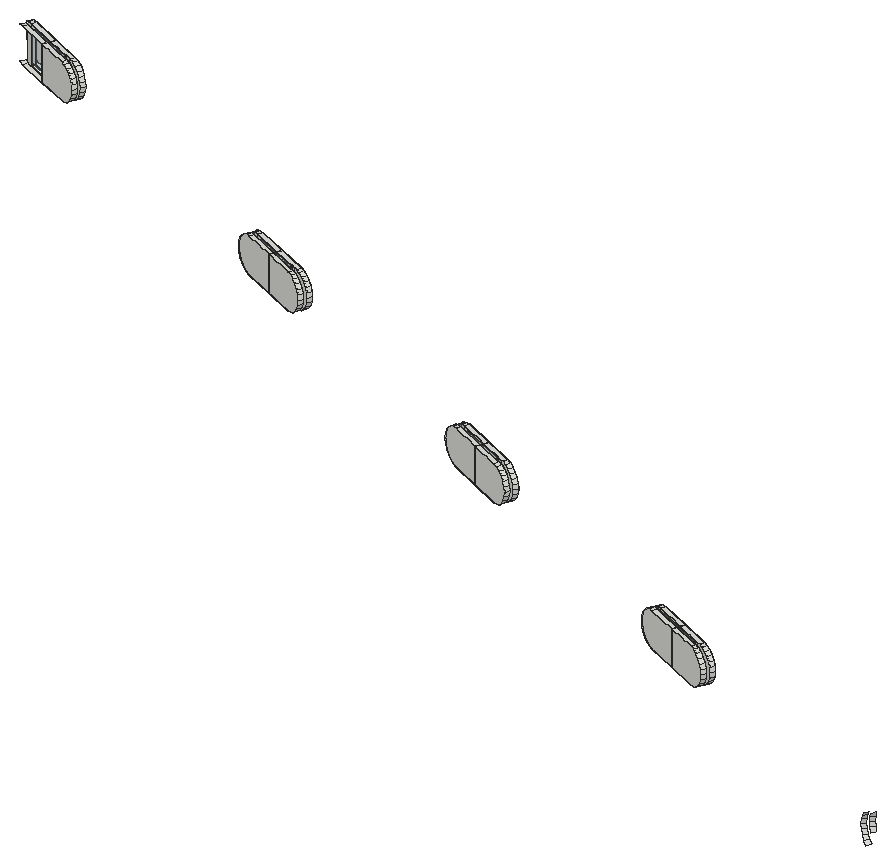
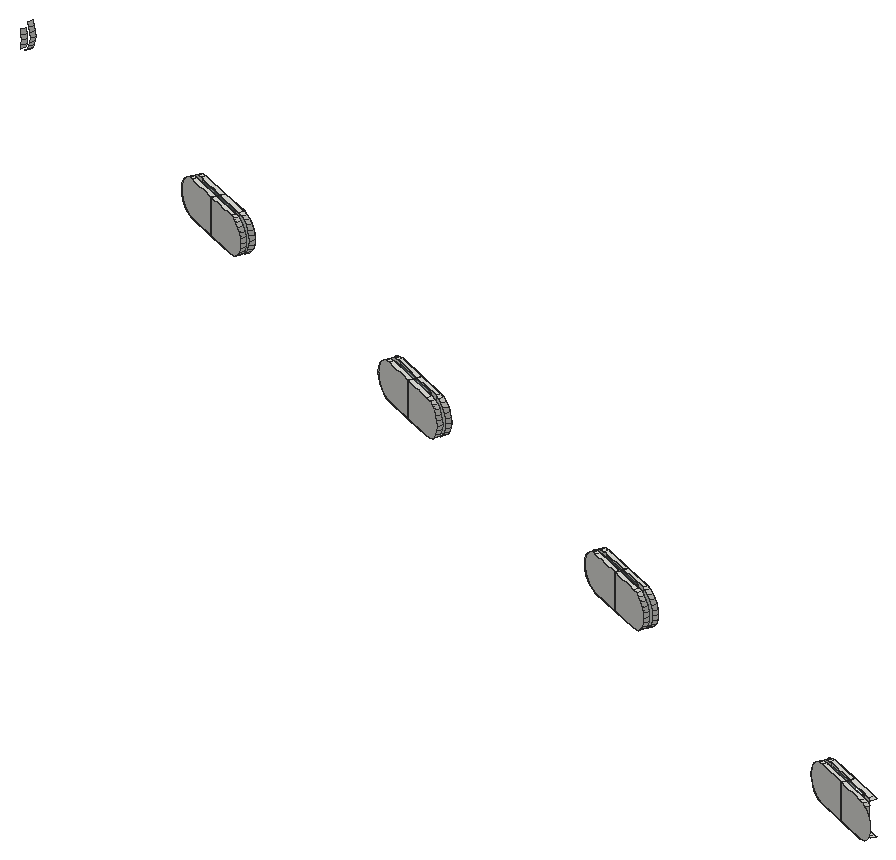
# SketchUp Ruby script. Lengths in inches.
U = 1.inch
M = Sketchup.active_model
def pt(a) = Geom::Point3d.new(a.map { |v| v * U })
def face(e, loops, mat)
  f = e.add_face(loops[0].map { |a| pt(a) })
  loops[1..].each { |l| e.add_face(l.map { |a| pt(a) }).erase! }
  f.material = f.back_material = mat if mat
  f
end
# faces: each face lists its corners as indices into pts; further lists are holes
def faces(e, pts, list, mat = nil) = list.each { |f| face(e, (f[0].is_a?(Array) ? f : [f]).map { |l| l.map { |i| pts[i] } }, mat) }
# xy, xz, yz: faces in a plane at the given z, y or x. An outline is a flat list of corners, or four numbers for a rectangle; further outlines are holes
def ring(l) = l.size == 4 ? [[l[0], l[1]], [l[2], l[1]], [l[2], l[3]], [l[0], l[3]]] : l.each_slice(2).to_a
def flat(e, list, mat, &to3) = list.each { |f| face(e, (f[0].is_a?(Array) ? f : [f]).map { |l| ring(l).map { |u, v| to3.(u, v) } }, mat) }
def xy(e, z, list, mat = nil) = flat(e, list, mat) { |x, y| [x, y, z] }
def xz(e, y, list, mat = nil) = flat(e, list, mat) { |x, z| [x, y, z] }
def yz(e, x, list, mat = nil) = flat(e, list, mat) { |y, z| [x, y, z] }
def lines(e, pts, list) = list.each { |a, b| e.add_line(pt(pts[a]), pt(pts[b])) }
# prism: a flat outline (further loops are holes) pulled along v
def prism(e, loops, v, mat = nil)
  f = face(e, loops, mat); d = Geom::Vector3d.new(v.map { |x| x * U })
  f.pushpull(f.normal.samedirection?(d) ? d.length : -d.length)
end
def box(e, o, s, mat = nil) = prism(e, [[o, [o[0] + s[0], o[1], o[2]], [o[0] + s[0], o[1] + s[1], o[2]], [o[0], o[1] + s[1], o[2]]]], [0, 0, s[2]], mat)
def at(x, y, z, deg = 0) = Geom::Transformation.translation(pt([x, y, z])) * Geom::Transformation.rotation(ORIGIN, Z_AXIS, deg.degrees)
def axes(o, x, y, z) = Geom::Transformation.new([*x, 0, *y, 0, *z, 0, *pt(o).to_a, 1])
def part(name) = M.definitions.add(name)
# library, detail: a bought-in or finely detailed component or shape, given as its bounding box
def library(name, o, s) = part(name).tap { |d| box(d.entities, o, s) }
def detail(e, o, s) = box(e.add_group.entities, o, s)
def put(e, d, t, mat = nil) = e.add_instance(d, t).tap { |i| i.material = mat if mat }
def group(e, t, mat = nil) = e.add_group.tap { |g| g.transformation = t; g.material = mat if mat }.entities
root = M.entities
M.materials.add("Glass_Safety_01").color = [204, 235, 244]
M.materials["Glass_Safety_01"].alpha = 0.1
xy(root,333,[[977.4375,1032.31,975.63,1033.09,975.74,1033.34,977.39,1032.63,977.55,1032.56],[977.625,1032.74,977.47,1032.81,975.82,1033.53,975.93,1033.78,977.73,1032.99],[975.63,1033.09,973.83,1033.88,973.9375,1034.13,975.74,1033.34],[975.82,1033.53,974.02,1034.3125,974.125,1034.5625,975.93,1033.78],[958.98,1040.34,957.18,1041.13,957.29,1041.38,958.91,1040.67,959.09,1040.6],
  [959.17,1040.78,958.99,1040.85,957.36,1041.5625,957.47,1041.82,959.28,1041.03],[957.18,1041.13,955.37,1041.92,955.48,1042.17,957.29,1041.38],[957.36,1041.5625,955.56,1042.35,955.67,1042.6,957.47,1041.82],[939.6,1048.79,937.79,1049.57,937.9,1049.82,939.54,1049.11,939.71,1049.04],[939.79,1049.22,939.62,1049.29,937.98,1050.01,938.09,1050.26,939.9,1049.47],
  [937.79,1049.57,935.99,1050.36,936.1,1050.61,937.9,1049.82],[937.98,1050.01,936.18,1050.79,936.29,1051.04,938.09,1050.26],[918.36,1058.03,916.56,1058.82,916.67,1059.07,918.32,1058.35,918.47,1058.29],[918.55,1058.47,918.4,1058.53,916.75,1059.25,916.86,1059.51,918.66,1058.72],[916.56,1058.82,914.75,1059.61,914.86,1059.86,916.67,1059.07],
  [916.75,1059.25,914.94,1060.04,915.05,1060.29,916.86,1059.51]])
xy(root,333.08,[[977.18,1032.72,975.74,1033.34,975.82,1033.53,977.26,1032.9],[975.74,1033.34,974.3,1033.97,974.375,1034.15,975.82,1033.53],[958.73,1040.75,957.29,1041.38,957.36,1041.5625,958.81,1040.93],[957.29,1041.38,955.84,1042.01,955.92,1042.19,957.36,1041.5625],[939.35,1049.2,937.9,1049.82,937.98,1050.01,939.42,1049.375],
  [937.9,1049.82,936.46,1050.45,936.54,1050.63,937.98,1050.01],[918.11,1058.44,916.67,1059.07,916.75,1059.25,918.19,1058.625],[916.67,1059.07,915.23,1059.7,915.3,1059.88,916.75,1059.25]],"Glass_Safety_01")
xy(root,335.05,[[977.18,1032.72,977.26,1032.9,975.82,1033.53,975.74,1033.34],[975.74,1033.34,975.82,1033.53,974.375,1034.15,974.3,1033.97],[958.73,1040.75,958.81,1040.93,957.36,1041.5625,957.29,1041.38],[957.29,1041.38,957.36,1041.5625,955.92,1042.19,955.84,1042.01],[939.35,1049.2,939.42,1049.375,937.98,1050.01,937.9,1049.82],
  [937.9,1049.82,937.98,1050.01,936.54,1050.63,936.46,1050.45],[918.11,1058.44,918.19,1058.625,916.75,1059.25,916.67,1059.07],[916.67,1059.07,916.75,1059.25,915.3,1059.88,915.23,1059.7]],"Glass_Safety_01")
xy(root,335.125,[[977.4375,1032.31,977.55,1032.56,977.39,1032.63,975.74,1033.34,975.63,1033.09],[977.625,1032.74,977.73,1032.99,975.93,1033.78,975.82,1033.53,977.47,1032.81],[975.63,1033.09,975.74,1033.34,973.9375,1034.13,973.83,1033.88],[975.82,1033.53,975.93,1033.78,974.125,1034.5625,974.02,1034.3125],[958.98,1040.34,959.09,1040.6,958.91,1040.67,957.29,1041.38,957.18,1041.13],
  [959.17,1040.78,959.28,1041.03,957.47,1041.82,957.36,1041.5625,958.99,1040.85],[957.18,1041.13,957.29,1041.38,955.48,1042.17,955.37,1041.92],[957.36,1041.5625,957.47,1041.82,955.67,1042.6,955.56,1042.35],[939.6,1048.79,939.71,1049.04,939.54,1049.11,937.9,1049.82,937.79,1049.57],[939.79,1049.22,939.9,1049.47,938.09,1050.26,937.98,1050.01,939.62,1049.29],
  [937.79,1049.57,937.9,1049.82,936.1,1050.61,935.99,1050.36],[937.98,1050.01,938.09,1050.26,936.29,1051.04,936.18,1050.79],[918.36,1058.03,918.47,1058.29,918.32,1058.35,916.67,1059.07,916.56,1058.82],[918.55,1058.47,918.66,1058.72,916.86,1059.51,916.75,1059.25,918.4,1058.53],[916.56,1058.82,916.67,1059.07,914.86,1059.86,914.75,1059.61],
  [916.75,1059.25,916.86,1059.51,915.05,1060.29,914.94,1060.04]])
p = [[977.4375,1032.31,335.125],[975.63,1033.09,335.125],[975.63,1033.09,333],[977.4375,1032.31,333],[977.6875,1032.2,333.04],[977.92,1032.09,333.14],
  [978.125,1032.01,333.3125],[978.28,1031.9375,333.53],[978.38,1031.9,333.79],[978.41,1031.88,334.0625],[978.38,1031.9,334.34],[978.28,1031.9375,334.59],
  [978.125,1032.01,334.8125],[977.92,1032.09,334.98],[977.6875,1032.2,335.09],[977.55,1032.56,333],[977.39,1032.63,333],[977.39,1032.63,335.125],
  [977.55,1032.56,335.125],[977.8,1032.45,335.09],[978.03,1032.35,334.98],[978.24,1032.26,334.8125],[978.39,1032.19,334.59],[978.49,1032.15,334.34],
  [978.52,1032.13,334.0625],[978.49,1032.15,333.79],[978.39,1032.19,333.53],[978.24,1032.26,333.3125],[978.03,1032.35,333.14],[977.8,1032.45,333.04],
  [977.625,1032.74,335.125],[977.47,1032.81,335.125],[977.47,1032.81,333],[977.625,1032.74,333],[977.875,1032.63,333.04],[978.11,1032.53,333.14],
  [978.3125,1032.4375,333.3125],[978.47,1032.37,333.53],[978.57,1032.33,333.79],[978.6,1032.31,334.0625],[978.57,1032.33,334.34],[978.47,1032.37,334.59],
  [978.3125,1032.4375,334.8125],[978.11,1032.53,334.98],[977.875,1032.63,335.09],[977.99,1032.88,333.04],[978.22,1032.78,333.14],[975.74,1033.34,335.125],
  [975.74,1033.34,333],[975.74,1033.34,333.08],[977.18,1032.72,333.08],[977.18,1032.72,335.05],[975.74,1033.34,335.05],[975.93,1033.78,335.125],
  [977.73,1032.99,335.125],[977.99,1032.88,335.09],[978.22,1032.78,334.98],[978.42,1032.69,334.8125],[978.58,1032.625,334.59],[978.68,1032.58,334.34],
  [978.71,1032.57,334.0625],[978.68,1032.58,333.79],[978.58,1032.625,333.53],[978.42,1032.69,333.3125],[977.73,1032.99,333],[975.93,1033.78,333],
  [975.82,1033.53,333],[975.82,1033.53,335.125],[975.82,1033.53,335.05],[977.26,1032.9,335.05],[977.26,1032.9,333.08],[975.82,1033.53,333.08],
  [973.83,1033.88,335.125],[973.57,1033.99,335.09],[973.34,1034.09,334.98],[973.14,1034.18,334.8125],[972.98,1034.25,334.59],[972.89,1034.29,334.34],
  [972.85,1034.3,334.0625],[972.89,1034.29,333.79],[972.98,1034.25,333.53],[973.14,1034.18,333.3125],[973.34,1034.09,333.14],[973.57,1033.99,333.04],
  [973.83,1033.88,333],[973.9375,1034.13,333],[973.9375,1034.13,335.125],[974.3,1033.97,335.05],[974.3,1033.97,333.08],[974.02,1034.3125,335.125],
  [974.02,1034.3125,333],[974.375,1034.15,333.08],[974.375,1034.15,335.05],[974.125,1034.5625,335.125],[974.125,1034.5625,333],[973.87,1034.67,333.04],
  [973.64,1034.78,333.14],[973.4375,1034.86,333.3125],[973.28,1034.93,333.53],[973.18,1034.97,333.79],[973.15,1034.99,334.0625],[973.18,1034.97,334.34],
  [973.28,1034.93,334.59],[973.4375,1034.86,334.8125],[973.64,1034.78,334.98],[973.87,1034.67,335.09],[973.68,1034.24,333.04],[973.45,1034.34,333.14],
  [973.68,1034.24,335.09],[973.45,1034.34,334.98],[973.25,1034.43,334.8125],[973.09,1034.5,334.59],[973,1034.54,334.34],[972.96,1034.56,334.0625],
  [973,1034.54,333.79],[973.09,1034.5,333.53],[973.25,1034.43,333.3125],[973.76,1034.42,333.04],[973.53,1034.52,333.14],[973.33,1034.61,333.3125],
  [973.17,1034.68,333.53],[973.07,1034.72,333.79],[973.04,1034.74,334.0625],[973.07,1034.72,334.34],[973.17,1034.68,334.59],[973.33,1034.61,334.8125],
  [973.53,1034.52,334.98],[973.76,1034.42,335.09],[958.98,1040.34,335.125],[957.18,1041.13,335.125],[957.18,1041.13,333],[958.98,1040.34,333],
  [959.23,1040.23,333.04],[959.47,1040.13,333.14],[959.67,1040.04,333.3125],[959.82,1039.98,333.53],[959.92,1039.93,333.79],[959.95,1039.92,334.0625],
  [959.92,1039.93,334.34],[959.82,1039.98,334.59],[959.67,1040.04,334.8125],[959.47,1040.13,334.98],[959.23,1040.23,335.09],[959.34,1040.49,333.04],
  [959.58,1040.38,333.14],[959.09,1040.6,333],[958.91,1040.67,333],[958.91,1040.67,335.125],[959.09,1040.6,335.125],[959.34,1040.49,335.09],
  [959.58,1040.38,334.98],[959.78,1040.3,334.8125],[959.93,1040.23,334.59],[960.03,1040.1875,334.34],[960.06,1040.17,334.0625],[960.03,1040.1875,333.79],
  [959.93,1040.23,333.53],[959.78,1040.3,333.3125],[959.17,1040.78,335.125],[958.99,1040.85,335.125],[958.99,1040.85,333],[959.17,1040.78,333],
  [959.42,1040.67,333.04],[959.66,1040.57,333.14],[959.86,1040.48,333.3125],[960.01,1040.41,333.53],[960.11,1040.37,333.79],[960.14,1040.35,334.0625],
  [960.11,1040.37,334.34],[960.01,1040.41,334.59],[959.86,1040.48,334.8125],[959.66,1040.57,334.98],[959.42,1040.67,335.09],[957.47,1041.82,335.125],
  [959.28,1041.03,335.125],[959.53,1040.92,335.09],[959.77,1040.82,334.98],[959.97,1040.73,334.8125],[960.12,1040.66,334.59],[960.22,1040.62,334.34],
  [960.25,1040.61,334.0625],[960.22,1040.62,333.79],[960.12,1040.66,333.53],[959.97,1040.73,333.3125],[959.77,1040.82,333.14],[959.53,1040.92,333.04],
  [959.28,1041.03,333],[957.47,1041.82,333],[957.29,1041.38,335.125],[957.29,1041.38,333],[957.29,1041.38,333.08],[958.73,1040.75,333.08],
  [958.73,1040.75,335.05],[957.29,1041.38,335.05],[957.36,1041.5625,333],[957.36,1041.5625,335.125],[957.36,1041.5625,335.05],[958.81,1040.93,335.05],
  [958.81,1040.93,333.08],[957.36,1041.5625,333.08],[955.37,1041.92,335.125],[955.12,1042.03,335.09],[954.88,1042.13,334.98],[954.68,1042.22,334.8125],
  [954.53,1042.28,334.59],[954.43,1042.33,334.34],[954.4,1042.34,334.0625],[954.43,1042.33,333.79],[954.53,1042.28,333.53],[954.68,1042.22,333.3125],
  [954.88,1042.13,333.14],[955.12,1042.03,333.04],[955.37,1041.92,333],[955.48,1042.17,333],[955.48,1042.17,335.125],[955.84,1042.01,335.05],
  [955.84,1042.01,333.08],[955.56,1042.35,335.125],[955.56,1042.35,333],[955.92,1042.19,333.08],[955.92,1042.19,335.05],[955.67,1042.6,335.125],
  [955.67,1042.6,333],[955.42,1042.71,333.04],[955.18,1042.8125,333.14],[954.98,1042.9,333.3125],[954.83,1042.97,333.53],[954.73,1043.01,333.79],
  [954.69,1043.03,334.0625],[954.73,1043.01,334.34],[954.83,1042.97,334.59],[954.98,1042.9,334.8125],[955.18,1042.8125,334.98],[955.42,1042.71,335.09],
  [955.23,1042.28,333.04],[954.99,1042.38,333.14],[955.23,1042.28,335.09],[954.99,1042.38,334.98],[954.79,1042.47,334.8125],[954.64,1042.54,334.59],
  [954.54,1042.58,334.34],[954.51,1042.59,334.0625],[954.54,1042.58,333.79],[954.64,1042.54,333.53],[954.79,1042.47,333.3125],[955.31,1042.46,333.04],
  [955.07,1042.5625,333.14],[954.87,1042.65,333.3125],[954.72,1042.72,333.53],[954.62,1042.76,333.79],[954.58,1042.77,334.0625],[954.62,1042.76,334.34],
  [954.72,1042.72,334.59],[954.87,1042.65,334.8125],[955.07,1042.5625,334.98],[955.31,1042.46,335.09],[939.6,1048.79,335.125],[937.79,1049.57,335.125],
  [937.79,1049.57,333],[939.6,1048.79,333],[939.85,1048.68,333.04],[940.08,1048.57,333.14],[940.29,1048.49,333.3125],[940.44,1048.42,333.53],
  [940.54,1048.375,333.79],[940.57,1048.36,334.0625],[940.54,1048.375,334.34],[940.44,1048.42,334.59],[940.29,1048.49,334.8125],[940.08,1048.57,334.98],
  [939.85,1048.68,335.09],[939.71,1049.04,333],[939.54,1049.11,333],[939.54,1049.11,335.125],[939.71,1049.04,335.125],[939.96,1048.93,335.09],
  [940.19,1048.83,334.98],[940.4,1048.74,334.8125],[940.55,1048.67,334.59],[940.65,1048.63,334.34],[940.68,1048.61,334.0625],[940.65,1048.63,333.79],
  [940.55,1048.67,333.53],[940.4,1048.74,333.3125],[940.19,1048.83,333.14],[939.96,1048.93,333.04],[939.79,1049.22,335.125],[939.62,1049.29,335.125],
  [939.62,1049.29,333],[939.79,1049.22,333],[940.04,1049.11,333.04],[940.27,1049.01,333.14],[940.47,1048.92,333.3125],[940.63,1048.85,333.53],
  [940.73,1048.81,333.79],[940.76,1048.79,334.0625],[940.73,1048.81,334.34],[940.63,1048.85,334.59],[940.47,1048.92,334.8125],[940.27,1049.01,334.98],
  [940.04,1049.11,335.09],[938.09,1050.26,335.125],[939.9,1049.47,335.125],[940.15,1049.36,335.09],[940.38,1049.26,334.98],[940.58,1049.17,334.8125],
  [940.74,1049.1,334.59],[940.84,1049.0625,334.34],[940.87,1049.05,334.0625],[940.84,1049.0625,333.79],[940.74,1049.1,333.53],[940.58,1049.17,333.3125],
  [940.38,1049.26,333.14],[940.15,1049.36,333.04],[939.9,1049.47,333],[938.09,1050.26,333],[937.9,1049.82,335.125],[937.9,1049.82,333],
  [937.9,1049.82,333.08],[939.35,1049.2,333.08],[939.35,1049.2,335.05],[937.9,1049.82,335.05],[937.98,1050.01,333],[937.98,1050.01,335.125],
  [937.98,1050.01,335.05],[939.42,1049.375,335.05],[939.42,1049.375,333.08],[937.98,1050.01,333.08],[935.99,1050.36,335.125],[935.74,1050.47,335.09],
  [935.5,1050.57,334.98],[935.3,1050.66,334.8125],[935.14,1050.73,334.59],[935.05,1050.77,334.34],[935.01,1050.78,334.0625],[935.05,1050.77,333.79],
  [935.14,1050.73,333.53],[935.3,1050.66,333.3125],[935.5,1050.57,333.14],[935.74,1050.47,333.04],[935.99,1050.36,333],[936.1,1050.61,333],
  [936.1,1050.61,335.125],[936.46,1050.45,335.05],[936.46,1050.45,333.08],[936.18,1050.79,335.125],[936.18,1050.79,333],[936.54,1050.63,333.08],
  [936.54,1050.63,335.05],[936.29,1051.04,335.125],[936.29,1051.04,333],[936.03,1051.15,333.04],[935.8,1051.26,333.14],[935.6,1051.34,333.3125],
  [935.44,1051.41,333.53],[935.34,1051.45,333.79],[935.3125,1051.47,334.0625],[935.34,1051.45,334.34],[935.44,1051.41,334.59],[935.6,1051.34,334.8125],
  [935.8,1051.26,334.98],[936.03,1051.15,335.09],[935.85,1050.72,333.04],[935.61,1050.82,333.14],[935.85,1050.72,335.09],[935.61,1050.82,334.98],
  [935.41,1050.91,334.8125],[935.25,1050.98,334.59],[935.16,1051.02,334.34],[935.12,1051.04,334.0625],[935.16,1051.02,333.79],[935.25,1050.98,333.53],
  [935.41,1050.91,333.3125],[935.92,1050.9,333.04],[935.6875,1051,333.14],[935.49,1051.09,333.3125],[935.33,1051.16,333.53],[935.23,1051.2,333.79],
  [935.2,1051.22,334.0625],[935.23,1051.2,334.34],[935.33,1051.16,334.59],[935.49,1051.09,334.8125],[935.6875,1051,334.98],[935.92,1050.9,335.09],
  [918.36,1058.03,335.125],[916.56,1058.82,335.125],[916.56,1058.82,333],[918.36,1058.03,333],[918.62,1057.92,333.04],[918.85,1057.82,333.14],
  [919.05,1057.73,333.3125],[919.21,1057.67,333.53],[919.3,1057.625,333.79],[919.34,1057.61,334.0625],[919.3,1057.625,334.34],[919.21,1057.67,334.59],
  [919.05,1057.73,334.8125],[918.85,1057.82,334.98],[918.62,1057.92,335.09],[918.73,1058.18,333.04],[918.96,1058.07,333.14],[918.47,1058.29,333],
  [918.32,1058.35,333],[918.32,1058.35,335.125],[918.47,1058.29,335.125],[918.73,1058.18,335.09],[918.96,1058.07,334.98],[919.16,1057.99,334.8125],
  [919.32,1057.92,334.59],[919.42,1057.875,334.34],[919.45,1057.86,334.0625],[919.42,1057.875,333.79],[919.32,1057.92,333.53],[919.16,1057.99,333.3125],
  [918.55,1058.47,335.125],[918.4,1058.53,335.125],[918.4,1058.53,333],[918.55,1058.47,333],[918.8,1058.36,333.04],[919.04,1058.25,333.14],
  [919.24,1058.17,333.3125],[919.4,1058.1,333.53],[919.49,1058.06,333.79],[919.53,1058.04,334.0625],[919.49,1058.06,334.34],[919.4,1058.1,334.59],
  [919.24,1058.17,334.8125],[919.04,1058.25,334.98],[918.8,1058.36,335.09],[916.86,1059.51,335.125],[918.66,1058.72,335.125],[918.91,1058.61,335.09],
  [919.15,1058.51,334.98],[919.35,1058.42,334.8125],[919.51,1058.35,334.59],[919.6,1058.31,334.34],[919.64,1058.3,334.0625],[919.6,1058.31,333.79],
  [919.51,1058.35,333.53],[919.35,1058.42,333.3125],[919.15,1058.51,333.14],[918.91,1058.61,333.04],[918.66,1058.72,333],[916.86,1059.51,333],
  [916.67,1059.07,335.125],[916.67,1059.07,333],[916.67,1059.07,333.08],[918.11,1058.44,333.08],[918.11,1058.44,335.05],[916.67,1059.07,335.05],
  [916.75,1059.25,333],[916.75,1059.25,335.125],[916.75,1059.25,335.05],[918.19,1058.625,335.05],[918.19,1058.625,333.08],[916.75,1059.25,333.08],
  [914.86,1059.86,333],[914.86,1059.86,335.125],[915.23,1059.7,335.05],[915.23,1059.7,333.08],[914.94,1060.04,335.125],[914.94,1060.04,333],
  [915.3,1059.88,333.08],[915.3,1059.88,335.05],[915.05,1060.29,335.125],[915.05,1060.29,333],[914.8,1060.4,333.04],[914.57,1060.5,333.14],
  [914.36,1060.59,333.3125],[914.21,1060.66,333.53],[914.11,1060.7,333.79],[914.08,1060.72,334.0625],[914.11,1060.7,334.34],[914.21,1060.66,334.59],
  [914.36,1060.59,334.8125],[914.57,1060.5,334.98],[914.8,1060.4,335.09],[914.61,1059.97,333.04],[914.75,1059.61,333],[914.5,1059.72,333.04],
  [914.69,1060.15,333.04],[993.83,1025.47,333.3125],[994.03,1025.38,333.14],[993.92,1025.125,333.14],[993.72,1025.21,333.3125],[993.67,1025.53,333.53],
  [993.56,1025.28,333.53],[993.58,1025.58,333.79],[993.47,1025.32,333.79],[993.75,1025.71,333.53],[993.66,1025.76,333.79],[993.77,1026.01,333.79],
  [993.86,1025.97,333.53],[993.54,1025.59,334.0625],[993.43,1025.34,334.0625],[993.62,1025.77,334.0625],[993.73,1026.02,334.0625],[993.58,1025.58,334.34],
  [993.47,1025.32,334.34],[993.66,1025.76,334.34],[993.77,1026.01,334.34],[993.67,1025.53,334.59],[993.56,1025.28,334.59],[993.75,1025.71,334.59],
  [993.86,1025.97,334.59],[993.83,1025.47,334.8125],[993.72,1025.21,334.8125],[914.46,1060.25,334.98],[914.69,1060.15,335.09],[914.61,1059.97,335.09],
  [914.5,1059.72,335.09],[914.75,1059.61,335.125]]
faces(root,p,[[0,1,2,3,4,5,6,7,8,9,10,11,12,13,14],[15,16,17,18,19,20,21,22,23,24,25,26,27,28,29],[29,28,5,4],[15,29,4,3],[30,31,32,33,34,35,36,37,38,39,40,41,42,43,44],[35,34,45,46],[47,17,16,48,49,50,51,52],[53,54,55,56,57,58,59,60,61,62,63,46,45,64,65],
  [34,33,64,45],[66,32,31,67,68,69,70,71],[1,72,73,74,75,76,77,78,79,80,81,82,83,84,2],[49,48,2,1,47,52],[48,85,86,47,52,87,88,49],[67,89,90,66,71,91,92,68],[66,71,68,67,53,65],[93,53,65,94,95,96,97,98,99,100,101,102,103,104,105],
  [106,85,84,83],[107,106,83,82],[90,117,95,94],[117,118,96,95],[128,129,130,131,132,133,134,135,136,137,138,139,140,141,142],[143,144,133,132],[145,146,147,148,149,150,151,152,153,154,155,156,157,144,143],[145,143,132,131],
  [158,159,160,161,162,163,164,165,166,167,168,169,170,171,172],[173,174,175,176,177,178,179,180,181,182,183,184,185,186,187],[163,162,185,184],[188,147,146,189,190,191,192,193],[162,161,186,185],[194,160,159,195,196,197,198,199],[129,200,201,202,203,204,205,206,207,208,209,210,211,212,130],[190,189,130,129,188,193],
  [189,213,214,188,193,215,216,190],[195,217,218,194,199,219,220,196],[194,199,196,195,173,187],[221,173,187,222,223,224,225,226,227,228,229,230,231,232,233],[234,213,212,211],[235,234,211,210],[218,245,223,222],[245,246,224,223],
  [256,257,258,259,260,261,262,263,264,265,266,267,268,269,270],[271,272,273,274,275,276,277,278,279,280,281,282,283,284,285],[285,284,261,260],[271,285,260,259],[286,287,288,289,290,291,292,293,294,295,296,297,298,299,300],[301,302,303,304,305,306,307,308,309,310,311,312,313,314,315],[291,290,313,312],[316,273,272,317,318,319,320,321],
  [290,289,314,313],[322,288,287,323,324,325,326,327],[257,328,329,330,331,332,333,334,335,336,337,338,339,340,258],[318,317,258,257,316,321],[317,341,342,316,321,343,344,318],[323,345,346,322,327,347,348,324],[322,327,324,323,301,315],[349,301,315,350,351,352,353,354,355,356,357,358,359,360,361],
  [362,341,340,339],[363,362,339,338],[346,373,351,350],[373,374,352,351],[384,385,386,387,388,389,390,391,392,393,394,395,396,397,398],[399,400,389,388],[401,402,403,404,405,406,407,408,409,410,411,412,413,400,399],[401,399,388,387],
  [414,415,416,417,418,419,420,421,422,423,424,425,426,427,428],[429,430,431,432,433,434,435,436,437,438,439,440,441,442,443],[419,418,441,440],[444,403,402,445,446,447,448,449],[418,417,442,441],[450,416,415,451,452,453,454,455],[446,445,386,385,444,449],[445,456,457,444,449,458,459,446],
  [451,460,461,450,455,462,463,452],[450,455,452,451,429,443],[464,429,443,465,466,467,468,469,470,471,472,473,474,475,476],[477,456,478,479],[461,480,466,465],[481,482,483,484],[28,27,6,5],[36,35,46,63],
  [116,107,82,81],[118,119,97,96],[144,157,134,133],[164,163,184,183],[244,235,210,209],[246,247,225,224],[284,283,262,261],[292,291,312,311],
  [372,363,338,337],[374,375,353,352],[400,413,390,389],[420,419,440,439],[485,481,484,486],[27,26,7,6],[37,36,63,62],[115,116,81,80],
  [119,120,98,97],[157,156,135,134],[165,164,183,182],[243,244,209,208],[247,248,226,225],[283,282,263,262],[293,292,311,310],[371,372,337,336],
  [375,376,354,353],[413,412,391,390],[421,420,439,438],[487,485,486,488],[489,490,491,492],[26,25,8,7],[38,37,62,61],[114,115,80,79],
  [120,121,99,98],[156,155,136,135],[166,165,182,181],[242,243,208,207],[248,249,227,226],[282,281,264,263],[294,293,310,309],[370,371,336,335],
  [376,377,355,354],[412,411,392,391],[422,421,438,437],[493,487,488,494],[490,495,496,491],[25,24,9,8],[39,38,61,60],[113,114,79,78],
  [121,122,100,99],[155,154,137,136],[167,166,181,180],[241,242,207,206],[249,250,228,227],[281,280,265,264],[295,294,309,308],[369,370,335,334],
  [377,378,356,355],[411,410,393,392],[423,422,437,436],[497,493,494,498],[495,499,500,496],[24,23,10,9],[40,39,60,59],[112,113,78,77],
  [122,123,101,100],[154,153,138,137],[168,167,180,179],[240,241,206,205],[250,251,229,228],[280,279,266,265],[296,295,308,307],[368,369,334,333],
  [378,379,357,356],[410,409,394,393],[424,423,436,435],[501,497,498,502],[499,503,504,500],[23,22,11,10],[41,40,59,58],[111,112,77,76],
  [123,124,102,101],[153,152,139,138],[169,168,179,178],[239,240,205,204],[251,252,230,229],[279,278,267,266],[297,296,307,306],[367,368,333,332],
  [379,380,358,357],[409,408,395,394],[425,424,435,434],[505,501,502,506],[22,21,12,11],[42,41,58,57],[110,111,76,75],[124,125,103,102],
  [152,151,140,139],[170,169,178,177],[238,239,204,203],[252,253,231,230],[278,277,268,267],[298,297,306,305],[366,367,332,331],[380,381,359,358],
  [408,407,396,395],[426,425,434,433],[21,20,13,12],[43,42,57,56],[109,110,75,74],[125,126,104,103],[151,150,141,140],[171,170,177,176],
  [237,238,203,202],[253,254,232,231],[277,276,269,268],[299,298,305,304],[365,366,331,330],[381,382,360,359],[407,406,397,396],[427,426,433,432],
  [20,19,14,13],[44,43,56,55],[108,109,74,73],[126,127,105,104],[150,149,142,141],[172,171,176,175],[236,237,202,201],[254,255,233,232],
  [276,275,270,269],[300,299,304,303],[364,365,330,329],[382,383,361,360],[406,405,398,397],[428,427,432,431],[507,508,476,475],[19,18,0,14],
  [30,44,55,54],[86,108,73,72],[127,89,93,105],[149,148,128,142],[158,172,175,174],[214,236,201,200],[255,217,221,233],[275,274,256,270],
  [286,300,303,302],[342,364,329,328],[383,345,349,361],[405,404,384,398],[414,428,431,430],[457,509,510,511],[508,460,464,476]])
faces(root,p,[[85,86,108,109,110,111,112,113,114,115,116,107,106],[89,90,117,118,119,120,121,122,123,124,125,126,127],[213,214,236,237,238,239,240,241,242,243,244,235,234],[217,218,245,246,247,248,249,250,251,252,253,254,255],[341,342,364,365,366,367,368,369,370,371,372,363,362],[345,346,373,374,375,376,377,378,379,380,381,382,383],[50,49,52,51],[70,69,51,50],
  [71,70,69,68],[49,88,87,52],[71,49,52,68],[91,71,68,92],[88,87,92,91],[191,190,193,192],[198,197,192,191],[199,198,197,196],
  [190,216,215,193],[199,190,193,196],[219,199,196,220],[216,215,220,219],[319,318,321,320],[326,325,320,319],[327,326,325,324],[318,344,343,321],
  [327,318,321,324],[347,327,324,348],[344,343,348,347],[447,446,449,448],[454,453,448,447],[455,454,453,452],[446,459,458,449],[455,446,449,452],
  [462,455,452,463],[459,458,463,462]],"Glass_Safety_01")
